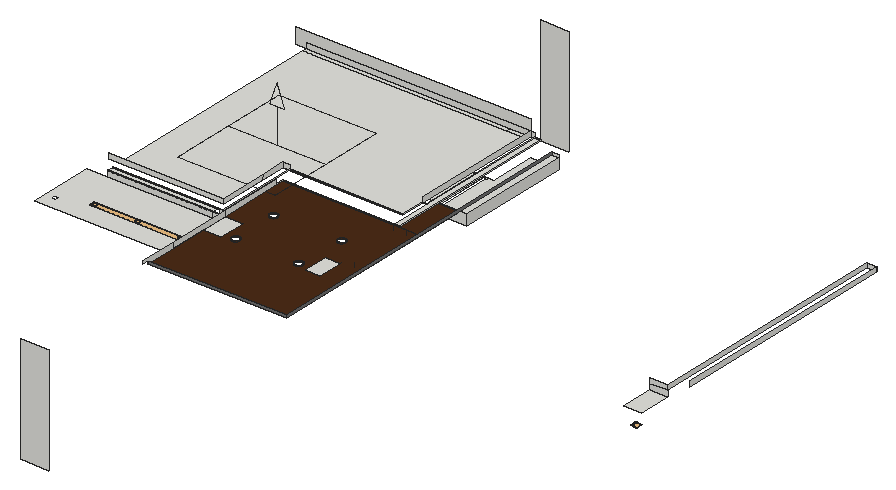
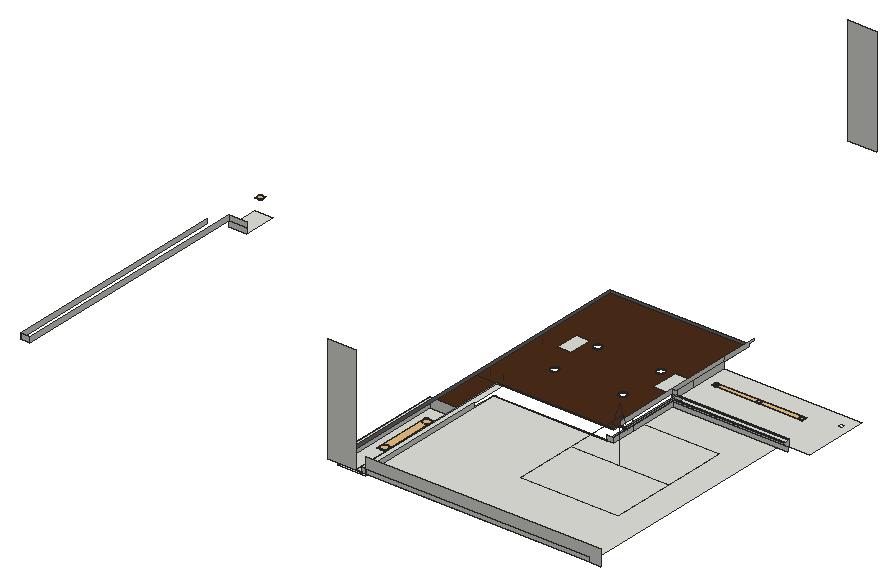
# SketchUp Ruby script. Lengths in inches.
U = 1.inch
M = Sketchup.active_model
def pt(a) = Geom::Point3d.new(a.map { |v| v * U })
def face(e, loops, mat)
  f = e.add_face(loops[0].map { |a| pt(a) })
  loops[1..].each { |l| e.add_face(l.map { |a| pt(a) }).erase! }
  f.material = f.back_material = mat if mat
  f
end
# faces: each face lists its corners as indices into pts; further lists are holes
def faces(e, pts, list, mat = nil) = list.each { |f| face(e, (f[0].is_a?(Array) ? f : [f]).map { |l| l.map { |i| pts[i] } }, mat) }
# xy, xz, yz: faces in a plane at the given z, y or x. An outline is a flat list of corners, or four numbers for a rectangle; further outlines are holes
def ring(l) = l.size == 4 ? [[l[0], l[1]], [l[2], l[1]], [l[2], l[3]], [l[0], l[3]]] : l.each_slice(2).to_a
def flat(e, list, mat, &to3) = list.each { |f| face(e, (f[0].is_a?(Array) ? f : [f]).map { |l| ring(l).map { |u, v| to3.(u, v) } }, mat) }
def xy(e, z, list, mat = nil) = flat(e, list, mat) { |x, y| [x, y, z] }
def xz(e, y, list, mat = nil) = flat(e, list, mat) { |x, z| [x, y, z] }
def yz(e, x, list, mat = nil) = flat(e, list, mat) { |y, z| [x, y, z] }
def lines(e, pts, list) = list.each { |a, b| e.add_line(pt(pts[a]), pt(pts[b])) }
# prism: a flat outline (further loops are holes) pulled along v
def prism(e, loops, v, mat = nil)
  f = face(e, loops, mat); d = Geom::Vector3d.new(v.map { |x| x * U })
  f.pushpull(f.normal.samedirection?(d) ? d.length : -d.length)
end
def box(e, o, s, mat = nil) = prism(e, [[o, [o[0] + s[0], o[1], o[2]], [o[0] + s[0], o[1] + s[1], o[2]], [o[0], o[1] + s[1], o[2]]]], [0, 0, s[2]], mat)
def at(x, y, z, deg = 0) = Geom::Transformation.translation(pt([x, y, z])) * Geom::Transformation.rotation(ORIGIN, Z_AXIS, deg.degrees)
def axes(o, x, y, z) = Geom::Transformation.new([*x, 0, *y, 0, *z, 0, *pt(o).to_a, 1])
def part(name) = M.definitions.add(name)
# library, detail: a bought-in or finely detailed component or shape, given as its bounding box
def library(name, o, s) = part(name).tap { |d| box(d.entities, o, s) }
def detail(e, o, s) = box(e.add_group.entities, o, s)
def put(e, d, t, mat = nil) = e.add_instance(d, t).tap { |i| i.material = mat if mat }
def group(e, t, mat = nil) = e.add_group.tap { |g| g.transformation = t; g.material = mat if mat }.entities
root = M.entities
M.materials.add("[Color M05]").color = [114, 114, 114]
M.materials.add("[Wood Veneer 01]").color = [76, 44, 23]
c1 = library("Group\#20",[-0.5,-0.5,-0.1],[139.5,7.875,0.2])
c2 = part("Group266\#1")
p = [[0,0,0],[0,0,-53.16],[-11.52,0,-53.16],[75.01,-97.09,0],[-75.01,-97.09,0],[75.01,97.09,0],
  [75.01,0,0],[-75.01,97.09,0],[11.52,0,-53.16],[-75.01,0,0],[0,0,-86.05]]
lines(c2.entities,p,[[0,1],[1,2],[3,4],[5,6],[7,5],[1,8],[9,0],[0,6],[8,10],[4,9],[6,3],[2,10],
  [9,7]])
c3 = part("Rectangle Light\#1")
put(c3.entities,c2,at(0,0,0))
c4 = library("Group\#22",[-0.5,-0.5,-0.1],[13.19,93.55,0.2])
c5 = library("Group\#26",[-0.5,-0.5,-0.1],[9.125,9.125,0.2])
xy(root,102.625,[[[2456.54,1821.9,2456.54,1844.2,2447.32,1844.2,2447.32,1928.83,2456.54,1928.83,2456.54,1998.71,2500.29,1998.71,2500.29,1821.9],[2481.48,1926.22,2483.06,1926.42,2484.53,1927.03,2485.79,1928,2486.76,1929.26,2487.37,1930.73,2487.57,1932.31,2487.37,1933.89,2486.76,1935.35,2485.79,1936.62,2484.53,1937.58,2483.06,1938.19,2481.48,1938.4,2479.9,1938.19,2478.44,1937.58,2477.17,1936.62,2476.21,1935.35,2475.6,1933.89,2475.39,1932.31,2475.6,1930.73,2476.21,1929.26,2477.17,1928,2478.44,1927.03,2479.9,1926.42],[2481.48,1845.85,2483.03,1846.05,2484.48,1846.65,2485.72,1847.61,2486.68,1848.85,2487.28,1850.3,2487.48,1851.85,2487.28,1853.4,2486.68,1854.85,2485.72,1856.09,2484.48,1857.05,2483.03,1857.65,2481.48,1857.85,2479.93,1857.65,2478.48,1857.05,2477.24,1856.09,2476.29,1854.85,2475.6875,1853.4,2475.48,1851.85,2475.6875,1850.3,2476.29,1848.85,2477.24,1847.61,2478.48,1846.65,2479.93,1846.05]],[2348.36,1844.2,2442.07,1928.14],[2442.07,1844.2,2442.76,1928.83],[2348.36,1928.14,2442.07,1928.83],[2442.76,1928.14,2443.44,1928.14,2443.44,1928.27,2447.32,1928.27,2447.32,1928.83,2442.76,1928.83],
  [2443.44,1928.14,2447.32,1928.27]])
xy(root,109.5,[[2930.51,1585.79,2957.51,1636.04]])
xy(root,109.625,[[[2064.92,1535.54,2276.89,1636.04],[2079.48,1553.19,2080.53,1553.33,2081.51,1553.73,2082.36,1554.38,2083,1555.22,2083.41,1556.2,2083.55,1557.25,2083.41,1558.3,2083,1559.28,2082.36,1560.125,2081.51,1560.77,2080.53,1561.18,2079.48,1561.31,2078.43,1561.18,2077.45,1560.77,2076.61,1560.125,2075.96,1559.28,2075.56,1558.3,2075.42,1557.25,2075.56,1556.2,2075.96,1555.22,2076.61,1554.38,2077.45,1553.73,2078.43,1553.33],[2127.54,1569.87,2128.43,1569.99,2129.26,1570.33,2129.97,1570.875,2130.52,1571.59,2130.86,1572.42,2130.98,1573.31,2130.86,1574.2,2130.52,1575.02,2129.97,1575.74,2129.26,1576.28,2128.43,1576.625,2127.54,1576.74,2126.65,1576.625,2125.82,1576.28,2125.11,1575.74,2124.5625,1575.02,2124.22,1574.2,2124.1,1573.31,2124.22,1572.42,2124.5625,1571.59,2125.11,1570.875,2125.82,1570.33,2126.65,1569.99],[2193.35,1569.87,2194.24,1569.99,2195.07,1570.33,2195.78,1570.875,2196.33,1571.59,2196.67,1572.42,2196.79,1573.31,2196.67,1574.2,2196.33,1575.02,2195.78,1575.74,2195.07,1576.28,2194.24,1576.625,2193.35,1576.74,2192.46,1576.625,2191.63,1576.28,2190.92,1575.74,2190.375,1575.02,2190.03,1574.2,2189.91,1573.31,2190.03,1572.42,2190.375,1571.59,2190.92,1570.875,2191.63,1570.33,2192.46,1569.99],[2259.16,1569.87,2260.05,1569.99,2260.88,1570.33,2261.6,1570.875,2262.14,1571.59,2262.48,1572.42,2262.6,1573.31,2262.48,1574.2,2262.14,1575.02,2261.6,1575.74,2260.88,1576.28,2260.05,1576.625,2259.16,1576.74,2258.27,1576.625,2257.45,1576.28,2256.73,1575.74,2256.1875,1575.02,2255.84,1574.2,2255.73,1573.31,2255.84,1572.42,2256.1875,1571.59,2256.73,1570.875,2257.45,1570.33,2258.27,1569.99]]])
xy(root,118.5,[[2276.89,1595.04,2304.32,1635.98],[2435.04,1595.04,2456.54,1632.6],[2097.23,1636.04,2258.0625,1645.27],[2097.23,1659.57,2097.23,2010.98,2440.84,2010.98,2440.84,1773.67,2256.86,1773.67,2256.86,1659.57],[2447.32,1746.92,2456.54,2018.36],
  [2489.98,1821.9,2500.29,1998.71],[2097.23,2010.98,2409.98,2018.36],[2409.98,2010.98,2440.84,2018.36]])
xy(root,118.5,[[[2276.89,1488.17,2276.89,1595.04,2304.32,1595.04,2304.32,1635.98,2276.89,1635.98,2276.89,1746.92,2489.98,1746.92,2489.98,1488.17],[2435.04,1595.04,2456.54,1632.6],[2321.71,1667.99,2323.26,1668.19,2324.71,1668.79,2325.95,1669.74,2326.91,1670.99,2327.5,1672.43,2327.71,1673.99,2327.5,1675.54,2326.91,1676.99,2325.95,1678.23,2324.71,1679.18,2323.26,1679.78,2321.71,1679.99,2320.16,1679.78,2318.71,1679.18,2317.47,1678.23,2316.51,1676.99,2315.91,1675.54,2315.71,1673.99,2315.91,1672.43,2316.51,1670.99,2317.47,1669.74,2318.71,1668.79,2320.16,1668.19],[2321.71,1595.24,2323.26,1595.44,2324.71,1596.04,2325.95,1596.99,2326.91,1598.24,2327.5,1599.68,2327.71,1601.24,2327.5,1602.79,2326.91,1604.24,2325.95,1605.48,2324.71,1606.43,2323.26,1607.03,2321.71,1607.24,2320.16,1607.03,2318.71,1606.43,2317.47,1605.48,2316.51,1604.24,2315.91,1602.79,2315.71,1601.24,2315.91,1599.68,2316.51,1598.24,2317.47,1596.99,2318.71,1596.04,2320.16,1595.44],[2418.52,1595.24,2420.07,1595.44,2421.52,1596.04,2422.76,1596.99,2423.72,1598.24,2424.32,1599.68,2424.52,1601.24,2424.32,1602.79,2423.72,1604.24,2422.76,1605.48,2421.52,1606.43,2420.07,1607.03,2418.52,1607.24,2416.97,1607.03,2415.52,1606.43,2414.28,1605.48,2413.33,1604.24,2412.73,1602.79,2412.52,1601.24,2412.73,1599.68,2413.33,1598.24,2414.28,1596.99,2415.52,1596.04,2416.97,1595.44],[2424.07,1671.22,2425.625,1671.43,2427.07,1672.03,2428.3125,1672.98,2429.27,1674.22,2429.87,1675.67,2430.07,1677.22,2429.87,1678.77,2429.27,1680.22,2428.3125,1681.46,2427.07,1682.42,2425.625,1683.02,2424.07,1683.22,2422.52,1683.02,2421.07,1682.42,2419.83,1681.46,2418.875,1680.22,2418.28,1678.77,2418.07,1677.22,2418.28,1675.67,2418.875,1674.22,2419.83,1672.98,2421.07,1672.03,2422.52,1671.43]],[2456.54,1746.92,2489.98,1821.9]],"[Wood Veneer 01]")
xz(root,1019,[[2456.54,118.5,2500.29,283.9375]])
xz(root,1488.17,[[2276.89,118.5,2489.98,122.875]],"[Color M05]")
xz(root,1636.04,[[2930.51,109.5,2957.51,118.5],[2097.23,109.625,2258.0625,118.5],[2258.0625,109.625,2276.89,118.5],[2097.23,118.5,2269.48,119.75],[2269.48,118.5,2276.89,126],
  [2930.51,118.5,2957.51,126]])
xz(root,1645.27,[[2097.23,118.5,2266.54,119.75]])
xz(root,1659.57,[[2079.65,118.5,2256.86,126]])
xz(root,1735.1,[[2269.48,118.5,2276.89,119.75]])
xz(root,1746.92,[[2276.89,118.5,2447.32,119.75],[2447.32,118.5,2456.54,119.75]])
xz(root,1773.67,[[2256.86,118.5,2266.54,126],[2266.54,118.5,2440.84,119.75]])
xz(root,1810.9,[[2440.84,118.5,2447.32,119.75]])
xz(root,1821.9,[[2456.54,102.625,2500.29,118.5]])
xz(root,1998.71,[[2489.98,118.5,2500.29,122.875]])
xz(root,2018.36,[[2079.65,118.5,2079.65,142.875,2440.84,142.875,2440.84,126,2097.23,126,2097.23,118.5],[2097.23,118.5,2440.84,126],[2440.84,118.5,2447.32,126],[2447.32,118.5,2456.54,119.75],[2456.54,118.5,2500.29,283.9375],
  [2957.51,118.5,2972.24,126]])
yz(root,2256.86,[[1659.57,118.5,1735.1,126],[1735.1,118.5,1773.67,126]])
yz(root,2266.54,[[1645.27,118.5,1773.67,119.75]])
yz(root,2269.48,[[1636.04,118.5,1735.1,119.75]])
yz(root,2276.89,[[1535.54,109.625,1595.04,118.5],[1595.04,109.625,1635.98,118.5],[1635.98,109.625,1636.04,118.5],[1488.17,118.5,1488.17,122.875,1478.85,122.875,1478.85,126,1535.54,126,1535.54,118.5],[1535.54,118.5,1636.04,126],
  [1636.04,118.5,1735.1,126],[1735.1,118.5,1746.92,119.75]])
yz(root,2440.84,[[1773.67,118.5,1810.9,119.75],[1810.9,118.5,2018.36,126]])
yz(root,2447.32,[[1810.9,118.5,2018.36,119.75]])
yz(root,2456.54,[[1746.92,118.5,2018.36,119.75]])
yz(root,2489.98,[[1488.17,118.5,1998.71,122.875]],"[Color M05]")
yz(root,2500.29,[[1821.9,102.625,1998.71,118.5]])
yz(root,2957.51,[[1636.04,118.5,2018.36,126]])
yz(root,2972.24,[[1659.57,118.5,2018.36,126]])
p = [[2481.48,1845.85,102.625],[2479.93,1846.05,102.625],[2479.93,1846.05,103.9375],[2481.48,1845.85,103.9375],[2483.03,1846.05,102.625],[2483.03,1846.05,103.9375],
  [2478.48,1846.65,102.625],[2478.48,1846.65,103.9375],[2484.48,1846.65,102.625],[2484.48,1846.65,103.9375],[2477.24,1847.61,102.625],[2477.24,1847.61,103.9375],
  [2485.72,1847.61,102.625],[2485.72,1847.61,103.9375],[2476.29,1848.85,102.625],[2476.29,1848.85,103.9375],[2486.68,1848.85,102.625],[2486.68,1848.85,103.9375],
  [2475.6875,1850.3,102.625],[2475.6875,1850.3,103.9375],[2487.28,1850.3,102.625],[2487.28,1850.3,103.9375],[2475.48,1851.85,102.625],[2475.48,1851.85,103.9375],
  [2487.48,1851.85,102.625],[2487.48,1851.85,103.9375],[2475.6875,1853.4,102.625],[2475.6875,1853.4,103.9375],[2487.28,1853.4,102.625],[2487.28,1853.4,103.9375],
  [2476.29,1854.85,102.625],[2476.29,1854.85,103.9375],[2486.68,1854.85,102.625],[2486.68,1854.85,103.9375],[2477.24,1856.09,102.625],[2477.24,1856.09,103.9375],
  [2485.72,1856.09,102.625],[2485.72,1856.09,103.9375],[2478.48,1857.05,102.625],[2478.48,1857.05,103.9375],[2484.48,1857.05,102.625],[2484.48,1857.05,103.9375],
  [2479.93,1857.65,102.625],[2479.93,1857.65,103.9375],[2483.03,1857.65,102.625],[2483.03,1857.65,103.9375],[2481.48,1857.85,102.625],[2481.48,1857.85,103.9375],
  [2481.48,1926.22,102.625],[2479.9,1926.42,102.625],[2479.9,1926.42,103.9375],[2481.48,1926.22,103.9375],[2483.06,1926.42,102.625],[2483.06,1926.42,103.9375],
  [2478.44,1927.03,102.625],[2478.44,1927.03,103.9375],[2484.53,1927.03,102.625],[2484.53,1927.03,103.9375],[2477.17,1928,102.625],[2477.17,1928,103.9375],
  [2485.79,1928,102.625],[2485.79,1928,103.9375],[2476.21,1929.26,102.625],[2476.21,1929.26,103.9375],[2486.76,1929.26,102.625],[2486.76,1929.26,103.9375],
  [2475.6,1930.73,102.625],[2475.6,1930.73,103.9375],[2487.37,1930.73,102.625],[2487.37,1930.73,103.9375],[2475.39,1932.31,102.625],[2475.39,1932.31,103.9375],
  [2487.57,1932.31,102.625],[2487.57,1932.31,103.9375],[2475.6,1933.89,102.625],[2475.6,1933.89,103.9375],[2487.37,1933.89,102.625],[2487.37,1933.89,103.9375],
  [2476.21,1935.35,102.625],[2476.21,1935.35,103.9375],[2486.76,1935.35,102.625],[2486.76,1935.35,103.9375],[2477.17,1936.62,102.625],[2477.17,1936.62,103.9375],
  [2485.79,1936.62,102.625],[2485.79,1936.62,103.9375],[2478.44,1937.58,102.625],[2478.44,1937.58,103.9375],[2484.53,1937.58,102.625],[2484.53,1937.58,103.9375],
  [2479.9,1938.19,102.625],[2479.9,1938.19,103.9375],[2483.06,1938.19,102.625],[2483.06,1938.19,103.9375],[2481.48,1938.4,102.625],[2481.48,1938.4,103.9375],
  [2972.07,1553.19,109.625],[2971.02,1553.33,109.625],[2971.02,1553.33,110.5625],[2972.07,1553.19,110.5625],[2970.04,1553.73,109.625],[2970.04,1553.73,110.5625],
  [2969.2,1554.38,109.625],[2969.2,1554.38,110.5625],[2968.55,1555.22,109.625],[2968.55,1555.22,110.5625],[2968.15,1556.2,109.625],[2968.15,1556.2,110.5625],
  [2968.01,1557.25,109.625],[2968.01,1557.25,110.5625],[2968.15,1558.3,109.625],[2968.15,1558.3,110.5625],[2968.55,1559.28,109.625],[2968.55,1559.28,110.5625],
  [2969.2,1560.125,109.625],[2969.2,1560.125,110.5625],[2970.04,1560.77,109.625],[2970.04,1560.77,110.5625],[2971.02,1561.18,109.625],[2971.02,1561.18,110.5625],
  [2972.07,1561.31,109.625],[2972.07,1561.31,110.5625],[2127.54,1569.87,109.625],[2126.65,1569.99,109.625],[2126.65,1569.99,110.0625],[2127.54,1569.87,110.0625],
  [2128.43,1569.99,109.625],[2128.43,1569.99,110.0625],[2193.35,1569.87,109.625],[2192.46,1569.99,109.625],[2192.46,1569.99,110.0625],[2193.35,1569.87,110.0625],
  [2194.24,1569.99,109.625],[2194.24,1569.99,110.0625],[2259.16,1569.87,109.625],[2258.27,1569.99,109.625],[2258.27,1569.99,110.0625],[2259.16,1569.87,110.0625],
  [2260.05,1569.99,109.625],[2260.05,1569.99,110.0625],[2125.82,1570.33,109.625],[2125.82,1570.33,110.0625],[2129.26,1570.33,109.625],[2129.26,1570.33,110.0625],
  [2191.63,1570.33,109.625],[2191.63,1570.33,110.0625],[2195.07,1570.33,109.625],[2195.07,1570.33,110.0625],[2257.45,1570.33,109.625],[2257.45,1570.33,110.0625],
  [2260.88,1570.33,109.625],[2260.88,1570.33,110.0625],[2125.11,1570.875,109.625],[2125.11,1570.875,110.0625],[2129.97,1570.875,109.625],[2129.97,1570.875,110.0625],
  [2190.92,1570.875,109.625],[2190.92,1570.875,110.0625],[2195.78,1570.875,109.625],[2195.78,1570.875,110.0625],[2256.73,1570.875,109.625],[2256.73,1570.875,110.0625],
  [2261.6,1570.875,109.625],[2261.6,1570.875,110.0625],[2124.5625,1571.59,109.625],[2124.5625,1571.59,110.0625],[2130.52,1571.59,109.625],[2130.52,1571.59,110.0625],
  [2190.375,1571.59,109.625],[2190.375,1571.59,110.0625],[2196.33,1571.59,109.625],[2196.33,1571.59,110.0625],[2256.1875,1571.59,109.625],[2256.1875,1571.59,110.0625],
  [2262.14,1571.59,109.625],[2262.14,1571.59,110.0625],[2124.22,1572.42,109.625],[2124.22,1572.42,110.0625],[2130.86,1572.42,109.625],[2130.86,1572.42,110.0625],
  [2190.03,1572.42,109.625],[2190.03,1572.42,110.0625],[2196.67,1572.42,109.625],[2196.67,1572.42,110.0625],[2255.84,1572.42,109.625],[2255.84,1572.42,110.0625],
  [2262.48,1572.42,109.625],[2262.48,1572.42,110.0625],[2124.1,1573.31,109.625],[2124.1,1573.31,110.0625],[2130.98,1573.31,109.625],[2130.98,1573.31,110.0625],
  [2189.91,1573.31,109.625],[2189.91,1573.31,110.0625],[2196.79,1573.31,109.625],[2196.79,1573.31,110.0625],[2255.73,1573.31,109.625],[2255.73,1573.31,110.0625],
  [2262.6,1573.31,109.625],[2262.6,1573.31,110.0625],[2124.22,1574.2,109.625],[2124.22,1574.2,110.0625],[2130.86,1574.2,109.625],[2130.86,1574.2,110.0625],
  [2190.03,1574.2,109.625],[2190.03,1574.2,110.0625],[2196.67,1574.2,109.625],[2196.67,1574.2,110.0625],[2255.84,1574.2,109.625],[2255.84,1574.2,110.0625],
  [2262.48,1574.2,109.625],[2262.48,1574.2,110.0625],[2124.5625,1575.02,109.625],[2124.5625,1575.02,110.0625],[2130.52,1575.02,109.625],[2130.52,1575.02,110.0625],
  [2190.375,1575.02,109.625],[2190.375,1575.02,110.0625],[2196.33,1575.02,109.625],[2196.33,1575.02,110.0625],[2256.1875,1575.02,109.625],[2256.1875,1575.02,110.0625],
  [2262.14,1575.02,109.625],[2262.14,1575.02,110.0625],[2125.11,1575.74,109.625],[2125.11,1575.74,110.0625],[2129.97,1575.74,109.625],[2129.97,1575.74,110.0625],
  [2190.92,1575.74,109.625],[2190.92,1575.74,110.0625],[2195.78,1575.74,109.625],[2195.78,1575.74,110.0625],[2256.73,1575.74,109.625],[2256.73,1575.74,110.0625],
  [2261.6,1575.74,109.625],[2261.6,1575.74,110.0625],[2125.82,1576.28,109.625],[2125.82,1576.28,110.0625],[2129.26,1576.28,109.625],[2129.26,1576.28,110.0625],
  [2191.63,1576.28,109.625],[2191.63,1576.28,110.0625],[2195.07,1576.28,109.625],[2195.07,1576.28,110.0625],[2257.45,1576.28,109.625],[2257.45,1576.28,110.0625],
  [2260.88,1576.28,109.625],[2260.88,1576.28,110.0625],[2126.65,1576.625,109.625],[2126.65,1576.625,110.0625],[2128.43,1576.625,109.625],[2128.43,1576.625,110.0625],
  [2192.46,1576.625,109.625],[2192.46,1576.625,110.0625],[2194.24,1576.625,109.625],[2194.24,1576.625,110.0625],[2258.27,1576.625,109.625],[2258.27,1576.625,110.0625],
  [2260.05,1576.625,109.625],[2260.05,1576.625,110.0625],[2127.54,1576.74,109.625],[2127.54,1576.74,110.0625],[2193.35,1576.74,109.625],[2193.35,1576.74,110.0625],
  [2259.16,1576.74,109.625],[2259.16,1576.74,110.0625],[2321.71,1595.24,118.5],[2320.16,1595.44,118.5],[2320.16,1595.44,119.375],[2321.71,1595.24,119.375],
  [2323.26,1595.44,118.5],[2323.26,1595.44,119.375],[2418.52,1595.24,118.5],[2416.97,1595.44,118.5],[2416.97,1595.44,119.375],[2418.52,1595.24,119.375],
  [2420.07,1595.44,118.5],[2420.07,1595.44,119.375],[2318.71,1596.04,118.5],[2318.71,1596.04,119.375],[2324.71,1596.04,118.5],[2324.71,1596.04,119.375],
  [2415.52,1596.04,118.5],[2415.52,1596.04,119.375],[2421.52,1596.04,118.5],[2421.52,1596.04,119.375],[2317.47,1596.99,118.5],[2317.47,1596.99,119.375],
  [2325.95,1596.99,118.5],[2325.95,1596.99,119.375],[2414.28,1596.99,118.5],[2414.28,1596.99,119.375],[2422.76,1596.99,118.5],[2422.76,1596.99,119.375],
  [2316.51,1598.24,118.5],[2316.51,1598.24,119.375],[2326.91,1598.24,118.5],[2326.91,1598.24,119.375],[2413.33,1598.24,118.5],[2413.33,1598.24,119.375],
  [2423.72,1598.24,118.5],[2423.72,1598.24,119.375],[2315.91,1599.68,118.5],[2315.91,1599.68,119.375],[2327.5,1599.68,118.5],[2327.5,1599.68,119.375],
  [2412.73,1599.68,118.5],[2412.73,1599.68,119.375],[2424.32,1599.68,118.5],[2424.32,1599.68,119.375],[2315.71,1601.24,118.5],[2315.71,1601.24,119.375],
  [2327.71,1601.24,118.5],[2327.71,1601.24,119.375],[2412.52,1601.24,118.5],[2412.52,1601.24,119.375],[2424.52,1601.24,118.5],[2424.52,1601.24,119.375],
  [2315.91,1602.79,118.5],[2315.91,1602.79,119.375],[2327.5,1602.79,118.5],[2327.5,1602.79,119.375],[2412.73,1602.79,118.5],[2412.73,1602.79,119.375],
  [2424.32,1602.79,118.5],[2424.32,1602.79,119.375],[2316.51,1604.24,118.5],[2316.51,1604.24,119.375],[2326.91,1604.24,118.5],[2326.91,1604.24,119.375],
  [2413.33,1604.24,118.5],[2413.33,1604.24,119.375],[2423.72,1604.24,118.5],[2423.72,1604.24,119.375],[2317.47,1605.48,118.5],[2317.47,1605.48,119.375],
  [2325.95,1605.48,118.5],[2325.95,1605.48,119.375],[2414.28,1605.48,118.5],[2414.28,1605.48,119.375],[2422.76,1605.48,118.5],[2422.76,1605.48,119.375],
  [2318.71,1606.43,118.5],[2318.71,1606.43,119.375],[2324.71,1606.43,118.5],[2324.71,1606.43,119.375],[2415.52,1606.43,118.5],[2415.52,1606.43,119.375],
  [2421.52,1606.43,118.5],[2421.52,1606.43,119.375],[2320.16,1607.03,118.5],[2320.16,1607.03,119.375],[2323.26,1607.03,118.5],[2323.26,1607.03,119.375],
  [2416.97,1607.03,118.5],[2416.97,1607.03,119.375],[2420.07,1607.03,118.5],[2420.07,1607.03,119.375],[2321.71,1607.24,118.5],[2321.71,1607.24,119.375],
  [2418.52,1607.24,118.5],[2418.52,1607.24,119.375],[2321.71,1667.99,118.5],[2320.16,1668.19,118.5],[2320.16,1668.19,119.375],[2321.71,1667.99,119.375],
  [2323.26,1668.19,118.5],[2323.26,1668.19,119.375],[2318.71,1668.79,118.5],[2318.71,1668.79,119.375],[2324.71,1668.79,118.5],[2324.71,1668.79,119.375],
  [2317.47,1669.74,118.5],[2317.47,1669.74,119.375],[2325.95,1669.74,118.5],[2325.95,1669.74,119.375],[2316.51,1670.99,118.5],[2316.51,1670.99,119.375],
  [2326.91,1670.99,118.5],[2326.91,1670.99,119.375],[2315.91,1672.43,118.5],[2315.91,1672.43,119.375],[2327.5,1672.43,118.5],[2327.5,1672.43,119.375],
  [2424.07,1671.22,118.5],[2422.52,1671.43,118.5],[2422.52,1671.43,119.375],[2424.07,1671.22,119.375],[2425.625,1671.43,118.5],[2425.625,1671.43,119.375],
  [2421.07,1672.03,118.5],[2421.07,1672.03,119.375],[2427.07,1672.03,118.5],[2427.07,1672.03,119.375],[2419.83,1672.98,118.5],[2419.83,1672.98,119.375],
  [2428.3125,1672.98,118.5],[2428.3125,1672.98,119.375],[2315.71,1673.99,118.5],[2315.71,1673.99,119.375],[2327.71,1673.99,118.5],[2327.71,1673.99,119.375],
  [2418.875,1674.22,118.5],[2418.875,1674.22,119.375],[2429.27,1674.22,118.5],[2429.27,1674.22,119.375],[2315.91,1675.54,118.5],[2315.91,1675.54,119.375],
  [2327.5,1675.54,118.5],[2327.5,1675.54,119.375],[2418.28,1675.67,118.5],[2418.28,1675.67,119.375],[2429.87,1675.67,118.5],[2429.87,1675.67,119.375],
  [2316.51,1676.99,118.5],[2316.51,1676.99,119.375],[2326.91,1676.99,118.5],[2326.91,1676.99,119.375],[2418.07,1677.22,118.5],[2418.07,1677.22,119.375],
  [2430.07,1677.22,118.5],[2430.07,1677.22,119.375],[2317.47,1678.23,118.5],[2317.47,1678.23,119.375],[2325.95,1678.23,118.5],[2325.95,1678.23,119.375],
  [2418.28,1678.77,118.5],[2418.28,1678.77,119.375],[2429.87,1678.77,118.5],[2429.87,1678.77,119.375],[2318.71,1679.18,118.5],[2318.71,1679.18,119.375],
  [2324.71,1679.18,118.5],[2324.71,1679.18,119.375],[2418.875,1680.22,118.5],[2418.875,1680.22,119.375],[2429.27,1680.22,118.5],[2429.27,1680.22,119.375],
  [2320.16,1679.78,118.5],[2320.16,1679.78,119.375],[2323.26,1679.78,118.5],[2323.26,1679.78,119.375],[2321.71,1679.99,118.5],[2321.71,1679.99,119.375],
  [2419.83,1681.46,118.5],[2419.83,1681.46,119.375],[2428.3125,1681.46,118.5],[2428.3125,1681.46,119.375],[2421.07,1682.42,118.5],[2421.07,1682.42,119.375],
  [2427.07,1682.42,118.5],[2427.07,1682.42,119.375],[2422.52,1683.02,118.5],[2422.52,1683.02,119.375],[2425.625,1683.02,118.5],[2425.625,1683.02,119.375],
  [2424.07,1683.22,118.5],[2424.07,1683.22,119.375],[2456.54,1635.98,118.5],[2456.54,1632.6,118.5],[2475.98,1636.04,118.5],[2475.98,1636.04,126],
  [2475.98,1635.98,118.5],[2475.98,1735.1,126],[2475.98,1735.1,118.5],[2456.54,1735.1,126],[2456.54,1735.1,118.5]]
faces(root,p,[[0,1,2,3],[4,0,3,5],[1,6,7,2],[8,4,5,9],[6,10,11,7],[12,8,9,13],[10,14,15,11],[16,12,13,17],
  [14,18,19,15],[20,16,17,21],[18,22,23,19],[24,20,21,25],[22,26,27,23],[28,24,25,29],[26,30,31,27],[32,28,29,33],
  [30,34,35,31],[36,32,33,37],[34,38,39,35],[40,36,37,41],[38,42,43,39],[44,40,41,45],[42,46,47,43],[46,44,45,47],
  [48,49,50,51],[52,48,51,53],[49,54,55,50],[56,52,53,57],[54,58,59,55],[60,56,57,61],[58,62,63,59],[64,60,61,65],
  [62,66,67,63],[68,64,65,69],[66,70,71,67],[72,68,69,73],[70,74,75,71],[76,72,73,77],[74,78,79,75],[80,76,77,81],
  [78,82,83,79],[84,80,81,85],[82,86,87,83],[88,84,85,89],[86,90,91,87],[92,88,89,93],[90,94,95,91],[94,92,93,95],
  [96,97,98,99],[97,100,101,98],[100,102,103,101],[102,104,105,103],[104,106,107,105],[106,108,109,107],[108,110,111,109],[110,112,113,111],
  [112,114,115,113],[114,116,117,115],[116,118,119,117],[118,120,121,119],[122,123,124,125],[126,122,125,127],[128,129,130,131],[132,128,131,133],
  [134,135,136,137],[138,134,137,139],[123,140,141,124],[142,126,127,143],[129,144,145,130],[146,132,133,147],[135,148,149,136],[150,138,139,151],
  [140,152,153,141],[154,142,143,155],[144,156,157,145],[158,146,147,159],[148,160,161,149],[162,150,151,163],[152,164,165,153],[166,154,155,167],
  [156,168,169,157],[170,158,159,171],[160,172,173,161],[174,162,163,175],[164,176,177,165],[178,166,167,179],[168,180,181,169],[182,170,171,183],
  [172,184,185,173],[186,174,175,187],[176,188,189,177],[190,178,179,191],[180,192,193,181],[194,182,183,195],[184,196,197,185],[198,186,187,199],
  [188,200,201,189],[202,190,191,203],[192,204,205,193],[206,194,195,207],[196,208,209,197],[210,198,199,211],[200,212,213,201],[214,202,203,215],
  [204,216,217,205],[218,206,207,219],[208,220,221,209],[222,210,211,223],[212,224,225,213],[226,214,215,227],[216,228,229,217],[230,218,219,231],
  [220,232,233,221],[234,222,223,235],[224,236,237,225],[238,226,227,239],[228,240,241,229],[242,230,231,243],[232,244,245,233],[246,234,235,247],
  [236,248,249,237],[250,238,239,251],[240,252,253,241],[254,242,243,255],[244,256,257,245],[258,246,247,259],[248,260,261,249],[260,250,251,261],
  [252,262,263,253],[262,254,255,263],[256,264,265,257],[264,258,259,265]])
faces(root,p,[[266,267,268,269],[270,266,269,271],[272,273,274,275],[276,272,275,277],[267,278,279,268],[280,270,271,281],[273,282,283,274],[284,276,277,285],
  [278,286,287,279],[288,280,281,289],[282,290,291,283],[292,284,285,293],[286,294,295,287],[296,288,289,297],[290,298,299,291],[300,292,293,301],
  [294,302,303,295],[304,296,297,305],[298,306,307,299],[308,300,301,309],[302,310,311,303],[312,304,305,313],[306,314,315,307],[316,308,309,317],
  [310,318,319,311],[320,312,313,321],[314,322,323,315],[324,316,317,325],[318,326,327,319],[328,320,321,329],[322,330,331,323],[332,324,325,333],
  [326,334,335,327],[336,328,329,337],[330,338,339,331],[340,332,333,341],[334,342,343,335],[344,336,337,345],[338,346,347,339],[348,340,341,349],
  [342,350,351,343],[352,344,345,353],[346,354,355,347],[356,348,349,357],[350,358,359,351],[358,352,353,359],[354,360,361,355],[360,356,357,361],
  [362,363,364,365],[366,362,365,367],[363,368,369,364],[370,366,367,371],[368,372,373,369],[374,370,371,375],[372,376,377,373],[378,374,375,379],
  [376,380,381,377],[382,378,379,383],[384,385,386,387],[388,384,387,389],[385,390,391,386],[392,388,389,393],[390,394,395,391],[396,392,393,397],
  [380,398,399,381],[400,382,383,401],[394,402,403,395],[404,396,397,405],[398,406,407,399],[408,400,401,409],[402,410,411,403],[412,404,405,413],
  [406,414,415,407],[416,408,409,417],[410,418,419,411],[420,412,413,421],[414,422,423,415],[424,416,417,425],[418,426,427,419],[428,420,421,429],
  [422,430,431,423],[432,424,425,433],[426,434,435,427],[436,428,429,437],[430,438,439,431],[440,432,433,441],[438,442,443,439],[442,440,441,443],
  [434,444,445,435],[446,436,437,447],[444,448,449,445],[450,446,447,451],[448,452,453,449],[454,450,451,455],[452,456,457,453],[456,454,455,457]],"[Wood Veneer 01]")
lines(root,p,[[458,459],[460,461],[460,462],[463,464],[465,466]])
put(root,c1,at(2124.1,1569.87,110.0625))
put(root,c3,axes([2216.51,1811.78,118.51],[1,0,0],[0,1,0],[0,0,-1]))
put(root,c4,at(2475.39,1845.85,103.9375))
put(root,c5,at(2968.01,1553.19,110.5625))
